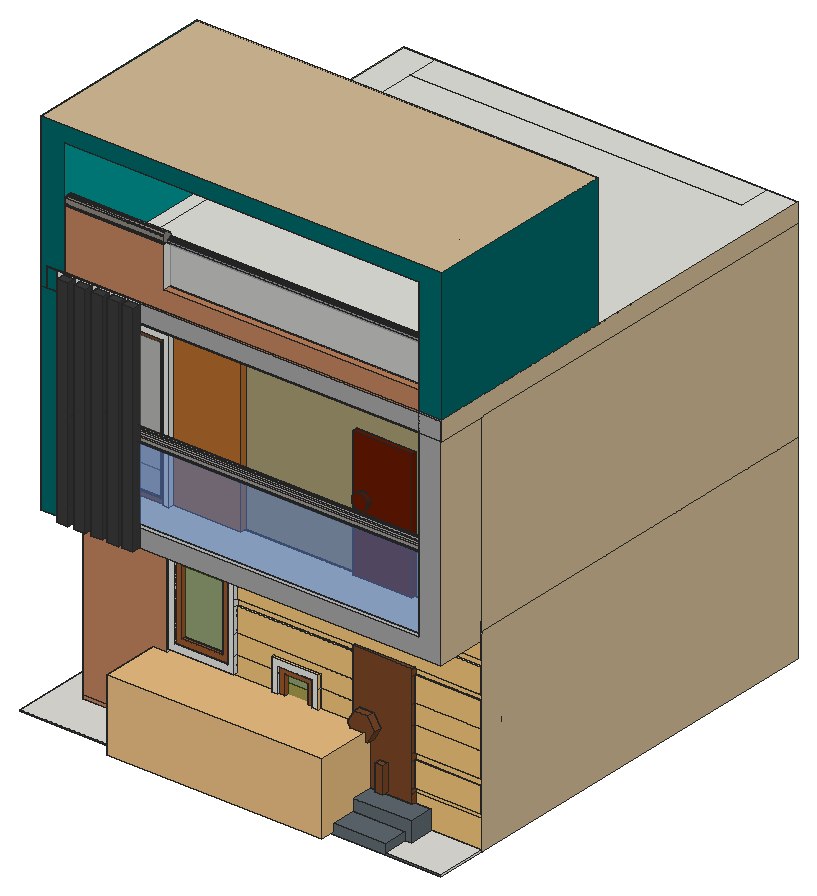
# SketchUp Ruby script. Lengths in inches.
U = 1.inch
M = Sketchup.active_model
def pt(a) = Geom::Point3d.new(a.map { |v| v * U })
def face(e, loops, mat)
  f = e.add_face(loops[0].map { |a| pt(a) })
  loops[1..].each { |l| e.add_face(l.map { |a| pt(a) }).erase! }
  f.material = f.back_material = mat if mat
  f
end
# faces: each face lists its corners as indices into pts; further lists are holes
def faces(e, pts, list, mat = nil) = list.each { |f| face(e, (f[0].is_a?(Array) ? f : [f]).map { |l| l.map { |i| pts[i] } }, mat) }
# xy, xz, yz: faces in a plane at the given z, y or x. An outline is a flat list of corners, or four numbers for a rectangle; further outlines are holes
def ring(l) = l.size == 4 ? [[l[0], l[1]], [l[2], l[1]], [l[2], l[3]], [l[0], l[3]]] : l.each_slice(2).to_a
def flat(e, list, mat, &to3) = list.each { |f| face(e, (f[0].is_a?(Array) ? f : [f]).map { |l| ring(l).map { |u, v| to3.(u, v) } }, mat) }
def xy(e, z, list, mat = nil) = flat(e, list, mat) { |x, y| [x, y, z] }
def xz(e, y, list, mat = nil) = flat(e, list, mat) { |x, z| [x, y, z] }
def yz(e, x, list, mat = nil) = flat(e, list, mat) { |y, z| [x, y, z] }
def lines(e, pts, list) = list.each { |a, b| e.add_line(pt(pts[a]), pt(pts[b])) }
# prism: a flat outline (further loops are holes) pulled along v
def prism(e, loops, v, mat = nil)
  f = face(e, loops, mat); d = Geom::Vector3d.new(v.map { |x| x * U })
  f.pushpull(f.normal.samedirection?(d) ? d.length : -d.length)
end
def box(e, o, s, mat = nil) = prism(e, [[o, [o[0] + s[0], o[1], o[2]], [o[0] + s[0], o[1] + s[1], o[2]], [o[0], o[1] + s[1], o[2]]]], [0, 0, s[2]], mat)
def at(x, y, z, deg = 0) = Geom::Transformation.translation(pt([x, y, z])) * Geom::Transformation.rotation(ORIGIN, Z_AXIS, deg.degrees)
def axes(o, x, y, z) = Geom::Transformation.new([*x, 0, *y, 0, *z, 0, *pt(o).to_a, 1])
def part(name) = M.definitions.add(name)
# library, detail: a bought-in or finely detailed component or shape, given as its bounding box
def library(name, o, s) = part(name).tap { |d| box(d.entities, o, s) }
def detail(e, o, s) = box(e.add_group.entities, o, s)
def put(e, d, t, mat = nil) = e.add_instance(d, t).tap { |i| i.material = mat if mat }
def group(e, t, mat = nil) = e.add_group.tap { |g| g.transformation = t; g.material = mat if mat }.entities
root = M.entities
M.materials.add("[Basic Tile]").color = [203, 206, 202]
M.materials.add("[Blacktop Old 01]").color = [132, 136, 139]
M.materials.add("[Color B08]").color = [102, 25, 0]
M.materials.add("[Color H07]").color = [0, 153, 153]
M.materials.add("[Color H08]").color = [0, 102, 102]
M.materials.add("[Color M07]").color = [58, 58, 58]
M.materials.add("[Concrete Aggregate Smoke]").color = [154, 150, 148]
M.materials.add("[Concrete Scored Jointless]").color = [140, 133, 127]
M.materials.add("[Concrete Tile]").color = [203, 190, 164]
M.materials.add("[Formica Beige]").color = [211, 187, 149]
M.materials.add("[Formica Speckled Grey]").color = [94, 105, 111]
M.materials.add("[Marble Carrara Gold Floor Tile]").color = [225, 223, 217]
M.materials.add("[Mirror 01]").color = [185, 185, 185]
M.materials.add("[Pavers Flagstone Gray]").color = [162, 162, 162]
M.materials.add("[Quartz Light Brown]").color = [199, 184, 152]
M.materials.add("[Terrazzo Light Blue]").color = [196, 214, 227]
M.materials.add("[Translucent Glass Blue]").color = [100, 149, 237]
M.materials["[Translucent Glass Blue]"].alpha = 0.5
M.materials.add("[Translucent Glass Dark Green]").color = [62, 91, 5]
M.materials["[Translucent Glass Dark Green]"].alpha = 0.5
M.materials.add("[Translucent Glass Gray]").color = [128, 128, 128]
M.materials["[Translucent Glass Gray]"].alpha = 0.5
M.materials.add("[Translucent Resin Crush Gray]").color = [184, 184, 184]
M.materials["[Translucent Resin Crush Gray]"].alpha = 0.8
M.materials.add("[Water Stream Shallow]").color = [155, 145, 133]
M.materials.add("[Wood Bamboo]").color = [177, 105, 43]
M.materials.add("[Wood Cherry Original]").color = [152, 86, 42]
M.materials.add("[Wood Floor Parquet]").color = [145, 89, 39]
M.materials.add("[Wood Lumber ButtJoined]").color = [164, 152, 112]
M.materials.add("[Wood OSB]").color = [240, 195, 122]
M.materials.add("[Wood Veneer 01]").color = [120, 70, 37]
M.materials.add("[Wood Veneer 02]").color = [190, 128, 91]
c1 = library("SHRUB",[-13.14,-8.45,-0.125],[75.37,32.45,24.02])
xy(root,0,[[0,4.95,16.1875,276],[16.1875,4.95,16.1875,276,16.63,276,16.63,32,67.83,32,67.83,35,180.1,35,180.1,33,216.1,33,216.1,36,256.1875,36,256.1875,4.95],[16.63,32,67.83,32,67.83,35,180.1,35,180.1,33,216.1,33,216.1,36,16.63,36],[16.63,36,256.1875,36,256.1875,244.95,247.63,244.95,247.63,45,25.63,45,25.63,244.95,16.63,244.95],[256.1875,36,256.1875,244.95,247.63,244.95,247.63,267,25.63,267,25.63,244.95,16.63,244.95,16.63,276,256.63,276,256.63,36],
  [25.63,45,247.63,244.95],[25.63,244.95,247.63,267]])
xy(root,1,[[173.84,20,173.84,35,180.1,35,180.1,33,216.1,33,216.1,35,226.28,35,226.28,20],[180.1,33,216.1,35]])
xy(root,1,[[0,4.95,173.84,4.95,173.84,35,67.83,35,67.83,32,16.63,32,16.63,276,0,276],[222.44,4.95,256.1875,4.95,256.1875,36,216.1,36,216.1,35,226.28,35,226.28,20,222.44,20]],"[Marble Carrara Gold Floor Tile]")
xy(root,3,[[16.63,32,67.83,36],[180.1,33,216.1,36],[67.83,35,151.74,36],[151.74,35,155.4,36],[155.4,35,159.06,36],
  [159.06,35,180.1,36],[67.83,36,151.74,39.4375],[151.74,36,155.4,39.4375],[155.4,36,159.06,39.4375],[159.06,36,180.1,39.4375]])
xy(root,6,[[173.84,4.95,222.44,20]],"[Formica Speckled Grey]")
xy(root,13,[[173.84,20,226.28,20,226.28,35,216.1,35,216.1,33,180.1,33,180.1,35,173.84,35]],"[Formica Speckled Grey]")
xy(root,14.41,[[196.71,29,201.46,33]])
xy(root,18.18,[[67.83,36,180.1,39.4375]])
xy(root,18.18,[[67.83,35,180.1,36]],"[Wood OSB]")
xy(root,19.49,[[130.75,33,159.06,36]],"[Wood OSB]")
xy(root,20.95,[[67.83,35,71.65,36],[71.65,35,75.54,36],[216.1,35,256.63,36],[159.06,36,180.1,40]])
xy(root,20.95,[[75.54,35,130.75,36],[159.06,35,180.1,36]],"[Wood OSB]")
xy(root,23.14,[[134.4,33,155.4,34],[134.4,34,155.4,36]])
xy(root,26.81,[[138.07,34,151.74,36]],"[Wood Cherry Original]")
xy(root,30.34,[[196.71,29,201.46,33]],"[Wood Veneer 01]")
xy(root,36.125,[[216.1,35,256.63,36],[159.06,36,180.1,40]])
xy(root,36.125,[[67.83,35,71.65,36],[71.65,35,75.54,36],[75.54,35,99.82,36],[99.82,35,100.35,36],[100.35,35,130.75,36],
  [159.06,35,180.1,36]],"[Wood OSB]")
xy(root,39.89,[[184.28,29,192.79,33]],"[Wood Veneer 01]")
xy(root,40.26,[[67.83,35,71.65,36],[71.65,35,75.54,36],[216.1,35,256.63,36]])
xy(root,40.26,[[75.54,35,130.75,36],[159.06,35,180.1,36]],"[Wood OSB]")
xy(root,45.68,[[67.83,33,108.0625,35],[67.83,35,108.0625,36]])
xy(root,49.49,[[71.65,33,104.25,34],[71.65,34,104.25,36]])
xy(root,53.39,[[75.54,34,100.35,36]],"[Wood Cherry Original]")
xy(root,54.64,[[184.28,29,192.79,33]],"[Wood Veneer 01]")
xy(root,55.4375,[[108.0625,35,130.75,36],[159.06,35,180.1,36],[216.1,35,256.63,36]])
xy(root,56.04,[[138.07,34,151.74,36]],"[Wood Cherry Original]")
xy(root,59.71,[[134.4,33,155.4,34],[134.4,34,155.4,36]])
xy(root,63.36,[[130.75,35,159.06,36]])
xy(root,63.36,[[130.75,33,159.06,35]],"[Wood OSB]")
xy(root,67.32,[[108.0625,35,180.1,36],[216.1,35,256.63,36]])
xy(root,82.5,[[108.0625,35,180.1,36],[216.1,35,256.63,36]])
xy(root,86.2,[[108.0625,35,180.1,36],[216.1,35,256.63,36]])
xy(root,87,[[180.1,35,216.1,36]])
xy(root,87,[[180.1,33,216.1,35]],"[Wood Veneer 01]")
xy(root,93.53,[[75.54,34,100.35,36]],"[Wood Cherry Original]")
xy(root,97.43,[[71.65,33,104.25,34],[71.65,34,104.25,36]])
xy(root,101.24,[[67.83,33,108.0625,35],[67.83,35,108.0625,36]])
xy(root,101.375,[[67.83,35,99.82,36],[99.82,35,180.1,36],[180.1,35,216.1,36],[216.1,35,256.63,36]])
xy(root,104.82,[[67.83,35,256.63,36]])
xy(root,114.54,[[72.76,5,256.15,35],[67.83,35,254.58,44]])
xy(root,114.54,[[36.83,0,36.83,5,12.82,5,12.82,32,67.83,32,67.83,35,72.76,35,72.76,5,43.69,5,43.69,0]],"[Color H07]")
xy(root,114.54,[[26.39,0,33.26,2],[47.39,0,54.26,5],[57.02,0,63.88,5],[65.89,0,72.76,5],[26.39,2,33.26,5]],"[Color M07]")
xy(root,117,[[25.63,45,247.63,267]])
xy(root,120,[[180.1,33,216.1,35],[67.83,35,99.82,36],[99.82,35,180.1,36],[180.1,35,216.1,36],[216.1,35,256.63,36]])
xy(root,125.64,[[25.76,5,36.83,8],[41.16,29,44.89,32],[67.83,29,71.5625,32],[44.89,30,67.83,32],[67.83,32,112.88,35],
  [67.83,35,112.88,36],[242.55,35,254.58,35.75],[254.58,35,256.15,35.75]])
xy(root,125.64,[[25.76,8,242.55,8,242.55,35,112.88,35,112.88,32,71.5625,32,71.5625,29,67.83,29,67.83,30,44.89,30,44.89,29,41.16,29,41.16,32,25.76,32],[112.88,35,242.55,35,242.55,35.75,254.58,35.75,254.58,44,67.83,44,67.83,36,112.88,36]],"[Basic Tile]")
xy(root,125.64,[[12.82,32,16.63,36]],"[Color H08]")
xy(root,125.64,[[43.69,5,242.55,8]],"[Mirror 01]")
xy(root,127.71,[[46.96,30,65.76,32]],"[Wood Veneer 01]")
xy(root,204,[[180.1,33,216.1,36]],"[Color B08]")
xy(root,213.66,[[46.96,30,65.76,32]],"[Wood Veneer 01]")
xy(root,215.73,[[44.89,29,67.83,30],[44.89,30,67.83,32]])
xy(root,219.46,[[41.16,29,71.5625,32]])
xy(root,236.32,[[12.82,5,22.32,8],[12.82,8,12.82,35.75,16.63,35.75,16.63,32,22.32,32,22.32,8],[16.63,32,22.32,35.75],[22.32,32,112.88,35.75],[12.82,35.75,16.63,36],
  [16.63,35.75,22.32,36],[22.32,35.75,112.88,36],[12.82,36,16.63,123.625],[16.63,36,22.32,123.625]])
xy(root,236.32,[[25.76,8,25.76,32,112.88,32,112.88,35.75,242.55,35.75,242.55,8]],"[Wood Floor Parquet]")
xy(root,237,[[16.63,5,25.76,36],[16.63,36,256.63,276]])
xy(root,237,[[26.39,5,99.82,36],[99.82,5,256.63,36]],"[Wood Floor Parquet]")
xy(root,237.45,[[25.76,5,26.39,36]])
xy(root,247.45,[[26.39,0,33.26,5],[36.83,0,43.69,8],[47.39,0,54.26,5],[57.02,0,63.88,5],[65.89,0,72.76,5]],"[Color M07]")
xy(root,248.02,[[16.63,5,22.32,8],[22.32,5,242.55,8],[242.55,5,256.15,8],[16.63,8,256.15,35.75],[16.63,35.75,22.32,123.625]])
xy(root,249,[[16.63,5,22.32,8],[22.32,5,27.38,8],[27.38,5,242.55,10.02],[242.55,5,256.63,123.6],[16.63,8,27.38,35.75],
  [27.38,10.02,237.59,10.02,237.59,24.04,35.67,24.04,35.67,121.625,27.38,121.625],[237.59,10.02,242.55,10.02,242.55,123.6,256.63,123.6,256.63,276,237.59,276,237.59,256.96,35.67,256.96,35.67,123.625,102.26,123.625,102.26,121.625,35.67,121.625,35.67,24.04,237.59,24.04],[16.63,35.75,22.32,123.625],[22.32,35.75,27.38,123.625],[27.38,121.625,35.67,123.625],
  [35.67,121.625,102.26,123.625],[16.63,123.625,35.67,276],[35.67,256.96,237.59,276]])
xy(root,260.27,[[87.26,5,242.55,10.02]],"[Wood Veneer 02]")
xy(root,285,[[27.38,5,87.26,7.13],[27.38,7.13,87.26,8],[87.26,7.64,242.55,10.02],[242.55,7.64,250.64,10.02],[27.38,8,87.26,10.02]])
xy(root,305.31,[[46.08,117.4375,84.2,120.4375],[46.08,120.4375,84.2,121.625]])
xy(root,306.9,[[47.67,120.4375,82.61,121.625]])
xy(root,306.9,[[47.67,117.4375,82.61,120.4375]],"[Terrazzo Light Blue]")
xy(root,312.03,[[47.67,117.4375,82.61,120.4375],[47.67,120.4375,82.61,121.625]])
xy(root,313.62,[[46.08,117.4375,84.2,120.4375],[46.08,120.4375,84.2,121.625]])
xy(root,319.63,[[27.38,121.625,102.26,123.625]])
xy(root,319.63,[[27.38,5,27.38,121.625,102.26,121.625,102.26,123.625,242.55,123.625,242.55,5]],"[Concrete Tile]")
xy(root,329.2,[[12.82,5,256.63,5,256.63,123.6,242.55,123.6,242.55,123.625,12.82,123.625]],"[Formica Beige]")
xz(root,0,[[26.39,114.54,33.26,247.45],[36.83,114.54,43.69,247.45],[47.39,114.54,54.26,247.45],[57.02,114.54,63.88,247.45],[65.89,114.54,72.76,247.45]],"[Color M07]")
xz(root,4.95,[[0,0,256.1875,0,256.1875,1,222.44,1,222.44,6,173.84,6,173.84,1,0,1]],"[Formica Speckled Grey]")
xz(root,5,[[26.39,114.54,33.26,125.64],[47.39,114.54,54.26,125.64],[57.02,114.54,63.88,125.64],[65.89,114.54,72.76,125.64],[26.39,125.64,33.26,237],
  [47.39,125.64,54.26,237],[57.02,125.64,63.88,237],[65.89,125.64,72.76,237],[22.32,237,25.76,237,25.76,237.45,26.39,237.45,26.39,247.45,33.26,247.45,33.26,237.45,72.76,237.45,72.76,248.02,22.32,248.02],[26.39,237,33.26,237.45],
  [33.26,237,36.83,237.45],[36.83,237,43.69,237.45],[43.69,237,47.39,237.45],[47.39,237,54.26,237.45],[54.26,237,57.02,237.45],
  [57.02,237,63.88,237.45],[63.88,237,65.89,237.45],[65.89,237,72.76,237.45],[72.76,237,242.55,237.45],[26.39,237.45,33.26,247.45],
  [26.39,237.45,33.26,247.45],[47.39,237.45,54.26,247.45],[57.02,237.45,63.88,247.45],[65.89,237.45,72.76,247.45]])
xz(root,5,[[12.82,114.54,26.39,114.54,26.39,125.64,25.76,125.64,25.76,237,22.32,237,22.32,236.32,12.82,236.32],[33.26,114.54,36.83,125.64],[43.69,114.54,47.39,125.64],[54.26,114.54,57.02,125.64],[63.88,114.54,65.89,125.64],
  [12.82,236.32,22.32,236.32,22.32,237,16.63,237,16.63,249,27.38,249,27.38,319.63,242.55,319.63,242.55,249,256.63,249,256.63,329.2,12.82,329.2],[16.63,237,22.32,248.02]],"[Color H08]")
xz(root,5,[[27.38,286.39,87.26,289.59]],"[Concrete Scored Jointless]")
xz(root,5,[[72.76,114.54,256.15,114.54,256.15,237,242.55,237,242.55,125.64,72.76,125.64],[242.55,237,256.15,248.02],[256.15,237,256.63,237,256.63,249,242.55,249,242.55,248.02,256.15,248.02],[72.76,237.45,242.55,248.02]],"[Pavers Flagstone Gray]")
xz(root,5,[[16.63,248.02,242.55,249],[27.38,249,242.55,249,242.55,260.27,87.26,260.27,87.26,285,27.38,285]],"[Wood Veneer 02]")
xz(root,8,[[36.83,125.64,43.69,139.27],[36.83,139.27,43.69,169.76],[36.83,169.76,43.69,170.73],[25.76,170.73,36.83,172.92],[36.83,170.73,43.69,172.92],
  [36.83,172.92,43.69,236.32],[36.83,236.32,43.69,247.45],[16.63,248.02,22.32,249]])
xz(root,8,[[25.76,125.64,36.83,169.76]],"[Color M07]")
xz(root,8,[[43.69,170.73,242.55,172.92]],"[Concrete Aggregate Smoke]")
xz(root,8,[[43.69,125.64,242.55,169.76]],"[Translucent Glass Blue]")
xz(root,10.02,[[27.38,249,27.38,285,87.26,285,87.26,260.27,237.59,260.27,237.59,249],[237.59,249,242.55,260.27],[242.55,282.625,250.64,285]])
xz(root,10.02,[[87.26,260.27,242.55,285]],"[Translucent Resin Crush Gray]")
xz(root,20,[[173.84,1,222.44,6]])
xz(root,20,[[222.44,1,226.28,1,226.28,13,173.84,13,173.84,6,222.44,6]],"[Formica Speckled Grey]")
xz(root,29,[[41.16,125.64,44.89,125.64,44.89,215.73,67.83,215.73,67.83,125.64,71.5625,125.64,71.5625,219.46,41.16,219.46]])
xz(root,29,[[196.71,14.41,201.46,30.34],[184.28,39.89,192.79,39.89,197.05,47.27,192.79,54.64,184.28,54.64,180.1,47.41,180.1,47.125]],"[Wood Veneer 01]")
xz(root,30,[[186.86,163.78,188.06,164.03,189.15,164.59,190.0625,165.4,190.73,166.43,191.11,167.59,191.18,168.81,190.93,170.01,190.38,171.1,189.5625,172.01,188.54,172.68,187.38,173.0625,186.16,173.13,184.96,172.88,183.87,172.33,182.95,171.51,182.28,170.49,181.9,169.33,181.83,168.11,182.08,166.91,182.63,165.82,183.45,164.9,184.47,164.23,185.64,163.85]],"[Color B08]")
xz(root,30,[[[44.89,125.64,67.83,215.73],[46.96,127.71,65.76,213.66]]],"[Wood Veneer 01]")
xz(root,32,[[16.63,0,67.83,1],[16.63,114.54,67.83,114.54,67.83,121.91,41.16,121.91,41.16,125.64,16.63,125.64],[41.16,121.91,67.83,125.64],[67.83,121.91,71.5625,125.64],[16.63,125.64,25.76,139.3125],
  [41.16,125.64,41.16,219.46,71.5625,219.46,71.5625,125.64,67.83,125.64,67.83,215.73,44.89,215.73,44.89,125.64],[[44.89,125.64,67.83,215.73],[46.96,127.71,65.76,213.66]],[16.63,139.3125,25.76,236.32]])
xz(root,32,[[12.82,114.54,16.63,125.64]],"[Color H08]")
xz(root,32,[[46.96,127.71,65.76,213.66]],"[Translucent Glass Gray]")
xz(root,32,[[25.76,125.64,41.16,125.64,41.16,219.46,71.5625,219.46,71.5625,125.64,112.88,125.64,112.88,236.32,25.76,236.32]],"[Wood Bamboo]")
xz(root,32,[[16.63,1,67.83,3],[16.63,3,67.83,114.54]],"[Wood Veneer 02]")
xz(root,33,[[180.1,0,216.1,1],[180.1,1,216.1,3],[180.1,3,216.1,13],[196.71,14.41,201.46,30.34],[[130.75,19.49,159.06,63.36],[134.4,23.14,155.4,59.71]],
  [184.28,39.89,180.1,47.125,180.1,47.41,184.28,54.64,192.79,54.64,197.05,47.27,192.79,39.89],[[67.83,45.68,108.0625,101.24],[71.65,49.49,104.25,97.43]],[180.1,47.125,180.1,47.41,180.02,47.27],[186.86,163.78,185.64,163.85,184.47,164.23,183.45,164.9,182.63,165.82,182.08,166.91,181.83,168.11,181.9,169.33,182.28,170.49,182.95,171.51,183.87,172.33,184.96,172.88,186.16,173.13,187.38,173.0625,188.54,172.68,189.5625,172.01,190.38,171.1,190.93,170.01,191.18,168.81,191.11,167.59,190.73,166.43,190.0625,165.4,189.15,164.59,188.06,164.03]])
xz(root,33,[[[180.1,120,216.1,204],[186.86,163.78,185.64,163.85,184.47,164.23,183.45,164.9,182.63,165.82,182.08,166.91,181.83,168.11,181.9,169.33,182.28,170.49,182.95,171.51,183.87,172.33,184.96,172.88,186.16,173.13,187.38,173.0625,188.54,172.68,189.5625,172.01,190.38,171.1,190.93,170.01,191.18,168.81,191.11,167.59,190.73,166.43,190.0625,165.4,189.15,164.59,188.06,164.03]]],"[Color B08]")
xz(root,33,[[[180.1,13,216.1,13,216.1,87,180.1,87,180.1,47.41,184.28,54.64,192.79,54.64,197.05,47.27,192.79,39.89,184.28,39.89,180.1,47.125],[196.71,14.41,201.46,30.34]]],"[Wood Veneer 01]")
xz(root,34,[[[134.4,23.14,155.4,59.71],[138.07,26.81,151.74,56.04]],[[71.65,49.49,104.25,97.43],[75.54,53.39,100.35,93.53]]],"[Wood Cherry Original]")
xz(root,35,[[67.83,0,151.74,1],[151.74,0,155.4,1],[155.4,0,159.06,1],[159.06,0,180.1,1],[173.84,1,180.1,3],
  [216.1,1,226.28,13],[173.84,3,180.1,13],[67.83,114.54,254.58,120],[254.58,114.54,256.15,120],[256.15,114.54,256.63,120],
  [67.83,120,254.58,125.64],[254.58,120,256.15,125.64]])
xz(root,35,[[67.83,1,173.84,3],[67.83,3,173.84,3,173.84,13,180.1,13,180.1,18.18,67.83,18.18],[67.83,20.95,130.75,36.125],[159.06,20.95,180.1,36.125],[216.1,20.95,256.63,36.125],
  [67.83,40.26,130.75,40.26,130.75,55.4375,108.0625,55.4375,108.0625,45.68,67.83,45.68],[159.06,40.26,180.1,55.4375],[216.1,40.26,256.63,55.4375],[108.0625,55.4375,130.75,55.4375,130.75,63.36,159.06,63.36,159.06,55.4375,180.1,55.4375,180.1,67.32,108.0625,67.32],[216.1,55.4375,256.63,67.32],
  [108.0625,67.32,180.1,82.5],[216.1,67.32,256.63,82.5],[108.0625,86.2,180.1,86.2,180.1,87,216.1,87,216.1,86.2,256.63,86.2,256.63,101.375,67.83,101.375,67.83,101.24,108.0625,101.24],[67.83,104.82,256.63,114.54]],"[Wood OSB]")
xz(root,35.75,[[242.55,125.64,242.55,236.32,22.32,236.32,22.32,248.02,256.15,248.02,256.15,125.64],[16.63,248.02,22.32,249]])
xz(root,36,[[16.63,0,216.1,3],[216.1,0,256.1875,1],[16.63,3,16.63,139.3125,112.88,139.3125,112.88,125.64,67.83,125.64,67.83,3],[67.83,3,180.1,18.18],[180.1,3,216.1,87],
  [[130.75,19.49,159.06,63.36],[134.4,23.14,155.4,59.71]],[67.83,20.95,130.75,36.125],[159.06,20.95,180.1,36.125],[216.1,20.95,256.63,36.125],[[134.4,23.14,155.4,59.71],[138.07,26.81,151.74,56.04]],
  [67.83,40.26,67.83,45.68,108.0625,45.68,108.0625,55.4375,130.75,55.4375,130.75,40.26],[159.06,40.26,180.1,55.4375],[216.1,40.26,256.63,55.4375],[[67.83,45.68,108.0625,101.24],[71.65,49.49,104.25,97.43]],[[71.65,49.49,104.25,97.43],[75.54,53.39,100.35,93.53]],
  [108.0625,55.4375,108.0625,67.32,180.1,67.32,180.1,55.4375,159.06,55.4375,159.06,63.36,130.75,63.36,130.75,55.4375],[216.1,55.4375,256.63,67.32],[108.0625,67.32,180.1,82.5],[216.1,67.32,256.63,82.5],[108.0625,86.2,108.0625,101.24,67.83,101.24,67.83,101.375,256.63,101.375,256.63,86.2,216.1,86.2,216.1,87,180.1,87,180.1,86.2],
  [67.83,104.82,256.63,120],[67.83,120,99.82,125.64],[180.1,120,216.1,204],[16.63,139.3125,112.88,236.32],[16.63,236.32,99.82,237],
  [25.76,237,26.39,237.45]])
xz(root,36,[[12.82,125.64,16.63,236.32]],"[Color H08]")
xz(root,36,[[138.07,26.81,151.74,56.04],[75.54,53.39,100.35,93.53]],"[Translucent Glass Dark Green]")
xz(root,36,[[99.82,120,180.1,120,180.1,204,216.1,204,216.1,120,256.63,120,256.63,237,99.82,237,99.82,236.32,112.88,236.32,112.88,125.64,99.82,125.64]],"[Wood Lumber ButtJoined]")
xz(root,36,[[256.1875,0,256.63,0,256.63,18.18,216.1,18.18,216.1,1,256.1875,1],[67.83,18.18,180.1,18.18,180.1,20.95,159.06,20.95,159.06,19.49,130.75,19.49,130.75,20.95,67.83,20.95],[216.1,18.18,256.63,20.95],[67.83,36.125,130.75,40.26],[159.06,36.125,180.1,40.26],
  [216.1,36.125,256.63,40.26],[108.0625,82.5,180.1,86.2],[216.1,82.5,256.63,86.2],[67.83,101.375,256.63,104.82]],"[Wood OSB]")
xz(root,39.4375,[[67.83,3,180.1,18.18]])
xz(root,40,[[159.06,20.95,180.1,36.125]])
xz(root,44,[[67.83,114.54,254.58,125.64]])
xz(root,45,[[25.63,0,247.63,117],[25.63,117,247.63,120],[25.63,120,247.63,237]])
xz(root,117.4375,[[[46.08,305.31,84.2,313.62],[47.67,306.9,82.61,312.03]]],"[Terrazzo Light Blue]")
xz(root,120.4375,[[[46.08,305.31,84.2,313.62],[47.67,306.9,82.61,312.03]]])
xz(root,121.625,[[[46.08,305.31,84.2,313.62],[47.67,306.9,82.61,312.03]]])
xz(root,121.625,[[[27.38,249,102.26,319.63],[46.08,305.31,84.2,313.62]]],"[Quartz Light Brown]")
xz(root,123.6,[[242.55,249,256.63,329.2]])
xz(root,123.625,[[12.82,236.32,12.82,329.2,27.38,329.2,27.38,249,16.63,249,16.63,248.02,22.32,248.02,22.32,236.32],[27.38,319.63,102.26,329.2],[102.26,319.63,242.55,329.2]])
xz(root,267,[[25.63,0,247.63,117],[25.63,117,247.63,120],[25.63,120,247.63,237]])
xz(root,276,[[0,0,16.63,1]])
xz(root,276,[[16.63,0,256.63,117],[16.63,117,256.63,120],[16.63,120,256.63,237],[16.63,237,256.63,249]],"[Formica Beige]")
yz(root,0,[[4.95,0,276,1]])
yz(root,12.82,[[5,114.54,5,236.32,36,236.32,36,125.64,32,125.64,32,114.54],[5,236.32,8,329.2],[8,236.32,35.75,329.2],[35.75,236.32,123.625,329.2]],"[Color H08]")
yz(root,16.63,[[32,0,36,1],[36,0,276,1],[32,1,36,3],[32,125.64,36,139.3125],[32,139.3125,36,236.32],
  [5,248.02,8,249],[8,248.02,35.75,249],[35.75,248.02,123.625,249]])
yz(root,16.63,[[36,1,276,237],[5,237,5,248.02,123.625,248.02,123.625,249,276,249,276,237]],"[Formica Beige]")
yz(root,16.63,[[32,3,36,125.64]],"[Wood Veneer 02]")
yz(root,22.32,[[5,236.32,8,248.02],[35.75,236.32,123.625,248.02]])
yz(root,25.63,[[45,0,267,117],[45,117,267,120],[45,120,267,237]])
yz(root,25.76,[[5,125.64,8,125.64,8,170.73,7.95,170.84,7.82,171.82,7.95,172.8125,8,172.92,8,236.32,6.2,237,5,237],[8,125.64,32,125.64,32,236.32,8,236.32,8,172.92,8.33,173.73,8.94,174.52,9.73,175.125,10.65,175.51,11.64,175.64,12.62,175.51,13.54,175.125,14.33,174.52,14.9375,173.73,15.32,172.8125,15.45,171.82,15.32,170.84,14.9375,169.92,14.33,169.13,13.54,168.52,12.62,168.14,11.64,168.01,10.65,168.14,9.73,168.52,8.94,169.13,8.33,169.92,8,170.73],[8,170.73,8,172.92,7.95,172.8125,7.82,171.82,7.95,170.84],[8,170.73,8,172.92,7.95,172.8125,7.82,171.82,7.95,170.84],[5,237,6.2,237,5,237.45],
  [6.2,237,36,237,36,237.45,5,237.45]])
yz(root,26.39,[[5,237,36,237.45]])
yz(root,26.39,[[0,114.54,5,247.45]],"[Color M07]")
yz(root,27.38,[[5,249,8,249,8,285,7.21,284.98,7.13,285,5,285],[8,249,10.02,285],[121.625,249,123.625,319.63],[7.21,284.98,8,285,7.13,285],[5,285,7.13,285,6.45,285.17,5.76,285.54,5.18,286.09,5,286.39],
  [5,286.39,5,289.59,4.72,289.07,4.53,288.3,4.55,287.51,4.77,286.76]])
yz(root,27.38,[[10.02,249,121.625,249,121.625,319.63,5,319.63,5,289.59,5.09,289.76,5.64,290.33,6.31,290.74,7.0625,290.96,7.85,290.98,8.62,290.8,9.31,290.42,9.88,289.875,10.29,289.2,10.51,288.45,10.53,287.66,10.35,286.9,9.97,286.2,9.43,285.63,8.76,285.22,8,285,10.02,285]],"[Color H07]")
yz(root,33.26,[[0,114.54,5,247.45]],"[Color M07]")
yz(root,36.83,[[5,125.64,8,139.27],[5,139.27,8,247.45]])
yz(root,36.83,[[0,114.54,5,139.27],[0,139.27,5,247.45]],"[Color M07]")
yz(root,41.16,[[29,125.64,32,219.46]])
yz(root,43.69,[[5,125.64,8,139.27],[5,139.27,8,247.45]])
yz(root,43.69,[[0,114.54,5,247.45]],"[Color M07]")
yz(root,44.89,[[29,125.64,30,215.73],[30,125.64,32,215.73]])
yz(root,46.08,[[117.4375,305.31,120.4375,313.62],[120.4375,305.31,121.625,313.62]])
yz(root,46.96,[[30,127.71,32,213.66]],"[Wood Veneer 01]")
yz(root,47.39,[[0,114.54,5,247.45]],"[Color M07]")
yz(root,47.67,[[117.4375,306.9,120.4375,312.03],[120.4375,306.9,121.625,312.03]])
yz(root,54.26,[[0,114.54,5,247.45]],"[Color M07]")
yz(root,57.02,[[0,114.54,5,247.45]],"[Color M07]")
yz(root,63.88,[[0,114.54,5,247.45]],"[Color M07]")
yz(root,65.76,[[30,127.71,32,213.66]],"[Wood Veneer 01]")
yz(root,65.89,[[0,114.54,5,247.45]],"[Color M07]")
yz(root,67.83,[[32,0,35,1],[32,1,35,3],[32,3,35,18.18],[35,3,36,18.18],[36,3,39.4375,18.18],
  [32,18.18,36,20.95],[32,20.95,35,36.125],[35,20.95,36,36.125],[32,36.125,36,40.26],[32,40.26,35,45.68],
  [35,40.26,36,45.68],[33,45.68,36,101.24],[35,101.24,36,101.375],[35,104.82,36,114.54],[32,114.54,35,125.64],
  [35,114.54,36,120],[36,114.54,44,125.64],[35,120,36,125.64],[29,125.64,30,215.73],[30,125.64,32,215.73]])
yz(root,67.83,[[32,45.68,33,45.68,33,101.24,35,101.24,35,101.375,36,101.375,36,104.82,35,104.82,35,114.54,32,114.54]],"[Wood Veneer 02]")
yz(root,71.5625,[[29,125.64,32,219.46]])
yz(root,71.65,[[33,49.49,34,97.43],[34,49.49,36,97.43]])
yz(root,72.76,[[0,114.54,5,247.45]],"[Color M07]")
yz(root,75.54,[[34,53.39,36,93.53]],"[Wood Cherry Original]")
yz(root,82.61,[[117.4375,306.9,120.4375,312.03],[120.4375,306.9,121.625,312.03]])
yz(root,84.2,[[117.4375,305.31,120.4375,313.62],[120.4375,305.31,121.625,313.62]])
yz(root,87.26,[[5,260.27,10.02,285],[10.02,282.625,10.02,285,8,285,8.76,285.22,9.43,285.63,9.97,286.2,10.35,286.9,10.45,287.32,10.63,287.29,11.2,287.06,11.7,286.68,12.07,286.1875,12.31,285.61,12.39,285,12.31,284.39,12.07,283.8125,11.7,283.32,11.2,282.94,10.63,282.71],[7.64,285,8,285,8.76,285.22,9.43,285.63,9.97,286.2,10.35,286.9,10.45,287.32,10.02,287.375,9.4,287.29,8.83,287.06,8.34,286.68,7.96,286.1875,7.72,285.61]])
yz(root,87.26,[[7.13,285,7.64,285,7.72,285.61,7.96,286.1875,8.34,286.68,8.83,287.06,9.4,287.29,10.02,287.375,10.45,287.32,10.53,287.66,10.51,288.45,10.29,289.2,9.88,289.875,9.31,290.42,8.62,290.8,7.85,290.98,7.0625,290.96,6.31,290.74,5.64,290.33,5.09,289.76,5,289.59,5,286.39,5.18,286.09,5.76,285.54,6.45,285.17]],"[Concrete Scored Jointless]")
yz(root,100.35,[[34,53.39,36,93.53]],"[Wood Cherry Original]")
yz(root,102.26,[[121.625,249,123.625,319.63]])
yz(root,104.25,[[33,49.49,34,97.43],[34,49.49,36,97.43]])
yz(root,108.0625,[[33,45.68,35,55.4375],[35,45.68,36,55.4375],[33,55.4375,35,67.32],[35,55.4375,36,67.32],[33,67.32,35,82.5],
  [35,67.32,36,82.5],[33,82.5,36,86.2],[33,86.2,35,101.24],[35,86.2,36,101.24]])
yz(root,112.88,[[32,125.64,36,236.32]],"[Wood Bamboo]")
yz(root,130.75,[[35,20.95,36,36.125],[35,40.26,36,55.4375],[35,55.4375,36,63.36]])
yz(root,130.75,[[33,19.49,36,20.95],[33,20.95,35,36.125],[33,36.125,36,40.26],[33,40.26,35,55.4375],[33,55.4375,35,63.36]],"[Wood OSB]")
yz(root,134.4,[[33,23.14,34,59.71],[34,23.14,36,59.71]])
yz(root,138.07,[[34,26.81,36,56.04]],"[Wood Cherry Original]")
yz(root,151.74,[[34,26.81,36,56.04]],"[Wood Cherry Original]")
yz(root,155.4,[[33,23.14,34,59.71],[34,23.14,36,59.71]])
yz(root,159.06,[[35,20.95,36,36.125],[36,20.95,40,36.125],[35,40.26,36,55.4375],[35,55.4375,36,63.36]])
yz(root,159.06,[[33,19.49,36,20.95],[33,20.95,35,36.125],[33,36.125,36,40.26],[33,40.26,35,55.4375],[33,55.4375,35,63.36]],"[Wood OSB]")
yz(root,173.84,[[4.95,1,20,6],[20,1,35,13]],"[Formica Speckled Grey]")
yz(root,180.1,[[33,0,35,1],[33,1,35,3],[33,3,35,13],[35,3,36,18.18],[36,3,39.4375,18.18],
  [35,20.95,36,36.125],[36,20.95,40,36.125],[35,40.26,36,55.4375],[35,55.4375,36,67.32],[35,67.32,36,82.5],
  [33,82.5,36,86.2],[33,86.2,35,87],[35,86.2,36,87]])
yz(root,180.1,[[33,120,36,204]],"[Color B08]")
yz(root,180.1,[[33,13,35,18.18],[33,18.18,36,20.95],[33,20.95,35,36.125],[33,36.125,36,40.26],[33,40.26,35,55.4375],
  [29,47.125,33,47.41],[33,55.4375,35,67.32],[33,67.32,35,82.5]],"[Wood Veneer 01]")
yz(root,196.71,[[29,14.41,33,30.34]],"[Wood Veneer 01]")
yz(root,201.46,[[29,14.41,33,30.34]],"[Wood Veneer 01]")
yz(root,216.1,[[33,0,36,1],[33,1,35,3],[35,1,36,3],[33,3,35,13],[35,20.95,36,36.125],
  [35,40.26,36,55.4375],[35,55.4375,36,67.32],[35,67.32,36,82.5],[35,86.2,36,87]])
yz(root,216.1,[[33,120,36,204]],"[Color B08]")
yz(root,216.1,[[35,3,36,3,36,18.18,33,18.18,33,13,35,13],[33,18.18,36,20.95],[33,20.95,35,36.125],[33,36.125,36,40.26],[33,40.26,35,55.4375],
  [33,55.4375,35,67.32],[33,67.32,35,82.5],[33,82.5,36,86.2],[33,86.2,35,87]],"[Wood Veneer 01]")
yz(root,222.44,[[4.95,1,20,6]],"[Formica Speckled Grey]")
yz(root,226.28,[[20,1,35,13]],"[Formica Speckled Grey]")
yz(root,242.55,[[5,249,10.02,260.27],[123.6,319.63,123.625,329.2]])
yz(root,242.55,[[[10.02,249,10.02,260.27,5,260.27,5,319.63,123.6,319.63,123.6,249],[10.02,282.625,10.63,282.71,11.2,282.94,11.7,283.32,12.07,283.8125,12.31,284.39,12.39,285,12.31,285.61,12.07,286.1875,11.7,286.68,11.2,287.06,10.63,287.29,10.02,287.375,9.4,287.29,8.83,287.06,8.34,286.68,7.96,286.1875,7.72,285.61,7.64,285,10.02,285]]],"[Color H07]")
yz(root,242.55,[[5,125.64,5,237.45,8,236.32,8,125.64],[8,125.64,8,170.73,8.33,169.92,8.94,169.13,9.73,168.52,10.65,168.14,11.64,168.01,12.62,168.14,13.54,168.52,14.33,169.13,14.9375,169.92,15.32,170.84,15.45,171.82,15.32,172.8125,14.9375,173.73,14.33,174.52,13.54,175.125,12.62,175.51,11.64,175.64,10.65,175.51,9.73,175.125,8.94,174.52,8.33,173.73,8,172.92,8,236.32,35.75,236.32,35.75,125.64]],"[Water Stream Shallow]")
yz(root,247.63,[[45,0,267,117],[45,117,267,120],[45,120,267,237]])
yz(root,250.64,[[10.02,282.625,10.02,285,7.64,285,7.72,285.61,7.96,286.1875,8.34,286.68,8.83,287.06,9.4,287.29,10.02,287.375,10.63,287.29,11.2,287.06,11.7,286.68,12.07,286.1875,12.31,285.61,12.39,285,12.31,284.39,12.07,283.8125,11.7,283.32,11.2,282.94,10.63,282.71]])
yz(root,254.58,[[35,114.54,44,125.64]])
yz(root,256.15,[[5,114.54,35,114.54,35,125.64,35.75,125.64,35.75,248.02,5,248.02]],"[Formica Beige]")
yz(root,256.1875,[[4.95,0,36,1]])
yz(root,256.63,[[35,20.95,36,36.125],[35,40.26,36,55.4375],[35,55.4375,36,67.32],[35,67.32,36,82.5],[35,86.2,36,101.375],
  [35,104.82,36,120]])
yz(root,256.63,[[5,249,123.6,329.2]],"[Color H08]")
yz(root,256.63,[[36,0,276,120],[36,120,276,237],[5,237,276,249]],"[Formica Beige]")
p = [[180.1,33,47.125],[184.28,33,39.89],[184.28,29,39.89],[180.1,29,47.125],[192.79,33,39.89],[197.05,33,47.27],
  [197.05,29,47.27],[192.79,29,39.89],[192.79,33,54.64],[192.79,29,54.64],[184.28,33,54.64],[180.1,33,47.41],
  [180.1,29,47.41],[184.28,29,54.64],[185.64,33,163.85],[186.86,33,163.78],[186.86,30,163.78],[185.64,30,163.85],
  [188.06,33,164.03],[188.06,30,164.03],[184.47,33,164.23],[184.47,30,164.23],[189.15,33,164.59],[189.15,30,164.59],
  [183.45,33,164.9],[183.45,30,164.9],[190.0625,33,165.4],[190.0625,30,165.4],[182.63,33,165.82],[182.63,30,165.82],
  [190.73,33,166.43],[190.73,30,166.43],[182.08,33,166.91],[182.08,30,166.91],[191.11,33,167.59],[191.11,30,167.59],
  [181.83,33,168.11],[181.83,30,168.11],[191.18,33,168.81],[191.18,30,168.81],[25.76,10.65,168.14],[25.76,11.64,168.01],
  [242.55,11.64,168.01],[242.55,10.65,168.14],[25.76,12.62,168.14],[242.55,12.62,168.14],[25.76,9.73,168.52],[242.55,9.73,168.52],
  [25.76,13.54,168.52],[242.55,13.54,168.52],[181.9,33,169.33],[181.9,30,169.33],[25.76,8.94,169.13],[242.55,8.94,169.13],
  [25.76,14.33,169.13],[242.55,14.33,169.13],[190.93,33,170.01],[190.93,30,170.01],[25.76,8.33,169.92],[242.55,8.33,169.92],
  [25.76,14.9375,169.92],[242.55,14.9375,169.92],[182.28,33,170.49],[182.28,30,170.49],[25.76,8,170.73],[242.55,8,170.73],
  [43.69,8,170.73],[36.83,8,170.73],[25.76,15.32,170.84],[242.55,15.32,170.84],[190.38,33,171.1],[190.38,30,171.1],
  [182.95,33,171.51],[182.95,30,171.51],[25.76,15.45,171.82],[242.55,15.45,171.82],[189.5625,33,172.01],[189.5625,30,172.01],
  [183.87,33,172.33],[183.87,30,172.33],[25.76,15.32,172.8125],[242.55,15.32,172.8125],[188.54,33,172.68],[188.54,30,172.68],
  [184.96,33,172.88],[184.96,30,172.88],[187.38,33,173.0625],[187.38,30,173.0625],[25.76,14.9375,173.73],[242.55,14.9375,173.73],
  [25.76,8.33,173.73],[25.76,8,172.92],[36.83,8,172.92],[43.69,8,172.92],[242.55,8,172.92],[242.55,8.33,173.73],
  [186.16,33,173.13],[186.16,30,173.13],[25.76,8.94,174.52],[242.55,8.94,174.52],[25.76,14.33,174.52],[242.55,14.33,174.52],
  [25.76,9.73,175.125],[242.55,9.73,175.125],[25.76,13.54,175.125],[242.55,13.54,175.125],[25.76,10.65,175.51],[242.55,10.65,175.51],
  [25.76,12.62,175.51],[242.55,12.62,175.51],[25.76,11.64,175.64],[242.55,11.64,175.64],[25.76,6.2,237],[25.76,8,236.32],
  [36.83,8,236.32],[43.69,8,236.32],[242.55,8,236.32],[242.55,5,237.45],[72.76,5,237.45],[65.89,5,237.45],
  [63.88,5,237.45],[57.02,5,237.45],[54.26,5,237.45],[47.39,5,237.45],[43.69,5,237.45],[36.83,5,237.45],
  [33.26,5,237.45],[26.39,5,237.45],[25.76,5,237.45],[242.55,10.63,282.71],[242.55,10.02,282.625],[250.64,10.02,282.625],
  [250.64,10.63,282.71],[87.26,10.63,282.71],[87.26,11.2,282.94],[242.55,11.2,282.94],[250.64,11.2,282.94],[87.26,11.7,283.32],
  [242.55,11.7,283.32],[250.64,11.7,283.32],[87.26,12.07,283.8125],[242.55,12.07,283.8125],[250.64,12.07,283.8125],[87.26,12.31,284.39],
  [242.55,12.31,284.39],[250.64,12.31,284.39],[87.26,12.39,285],[242.55,12.39,285],[250.64,12.39,285],[27.38,6.45,285.17],
  [27.38,7.13,285],[87.26,7.13,285],[87.26,6.45,285.17],[87.26,7.72,285.61],[87.26,7.64,285],[242.55,7.64,285],
  [242.55,7.72,285.61],[250.64,7.72,285.61],[250.64,7.64,285],[27.38,8,285],[27.38,8.76,285.22],[87.26,8.76,285.22],
  [87.26,8,285],[87.26,12.31,285.61],[242.55,12.31,285.61],[250.64,12.31,285.61],[27.38,5.76,285.54],[87.26,5.76,285.54],
  [27.38,9.43,285.63],[87.26,9.43,285.63],[27.38,5.18,286.09],[87.26,5.18,286.09],[87.26,7.96,286.1875],[242.55,7.96,286.1875],
  [250.64,7.96,286.1875],[27.38,9.97,286.2],[87.26,9.97,286.2],[87.26,12.07,286.1875],[242.55,12.07,286.1875],[250.64,12.07,286.1875],
  [27.38,5,286.39],[87.26,5,286.39],[87.26,8.34,286.68],[242.55,8.34,286.68],[250.64,8.34,286.68],[27.38,10.35,286.9],
  [87.26,10.35,286.9],[87.26,11.7,286.68],[242.55,11.7,286.68],[250.64,11.7,286.68],[87.26,8.83,287.06],[242.55,8.83,287.06],
  [250.64,8.83,287.06],[87.26,11.2,287.06],[242.55,11.2,287.06],[250.64,11.2,287.06],[27.38,10.53,287.66],[87.26,10.53,287.66],
  [87.26,10.45,287.32],[87.26,9.4,287.29],[242.55,9.4,287.29],[250.64,9.4,287.29],[87.26,10.63,287.29],[242.55,10.63,287.29],
  [250.64,10.63,287.29],[87.26,10.02,287.375],[242.55,10.02,287.375],[250.64,10.02,287.375],[27.38,10.51,288.45],[87.26,10.51,288.45],
  [27.38,10.29,289.2],[87.26,10.29,289.2],[27.38,9.88,289.875],[87.26,9.88,289.875],[27.38,5.09,289.76],[27.38,5,289.59],
  [87.26,5,289.59],[87.26,5.09,289.76],[27.38,5.64,290.33],[87.26,5.64,290.33],[27.38,9.31,290.42],[87.26,9.31,290.42],
  [27.38,6.31,290.74],[87.26,6.31,290.74],[27.38,8.62,290.8],[87.26,8.62,290.8],[27.38,7.0625,290.96],[87.26,7.0625,290.96],
  [27.38,7.85,290.98],[87.26,7.85,290.98],[315.04,-22.41,117],[315.04,-22.41,120],[26.39,2,125.64],[33.26,2,125.64],
  [242.55,35.75,319.63],[242.55,35.75,329.2]]
faces(root,p,[[0,1,2,3],[4,5,6,7],[5,8,9,6],[10,11,12,13]],"[Wood Veneer 01]")
faces(root,p,[[14,15,16,17],[15,18,19,16],[20,14,17,21],[18,22,23,19],[24,20,21,25],[22,26,27,23],[28,24,25,29],[26,30,31,27],
  [32,28,29,33],[30,34,35,31],[36,32,33,37],[34,38,39,35],[50,36,37,51],[38,56,57,39],[62,50,51,63],[56,70,71,57],
  [72,62,63,73],[70,76,77,71],[78,72,73,79],[76,82,83,77],[84,78,79,85],[82,86,87,83],[96,84,85,97],[86,96,97,87]],"[Color B08]")
faces(root,p,[[40,41,42,43],[41,44,45,42],[46,40,43,47],[44,48,49,45],[52,46,47,53],[48,54,55,49],[58,52,53,59],[54,60,61,55],
  [64,58,59,65,66,67],[60,68,69,61],[68,74,75,69],[74,80,81,75],[80,88,89,81],[90,91,92,93,94,95],[98,90,95,99],[88,100,101,89],
  [102,98,99,103],[100,104,105,101],[106,102,103,107],[104,108,109,105],[110,106,107,111],[108,110,111,109]],"[Concrete Aggregate Smoke]")
faces(root,p,[[112,113,114,115,116,117,118,119,120,121,122,123,124,125,126,127,128]],"[Wood Floor Parquet]")
faces(root,p,[[129,130,131,132],[135,129,132,136],[138,135,136,139],[141,138,139,142],[144,141,142,145],[147,144,145,148],[155,156,157,158],[164,147,148,165],
  [156,173,174,157],[178,164,165,179],[173,183,184,174],[188,178,179,189],[183,191,192,184],[194,188,189,195],[191,200,201,192],[203,194,195,204],
  [200,206,207,201],[206,203,204,207]])
faces(root,p,[[133,134,135,129],[134,137,138,135],[137,140,141,138],[140,143,144,141],[143,146,147,144],[153,154,155,156],[146,163,164,147],[172,153,156,173],
  [163,177,178,164],[182,172,173,183],[177,187,188,178],[190,182,183,191],[187,193,194,188],[199,190,191,200],[193,202,203,194],[205,199,200,206],
  [198,205,206,203,202]],"[Blacktop Old 01]")
faces(root,p,[[149,150,151,152],[159,160,161,162],[166,149,152,167],[160,168,169,161],[170,166,167,171],[168,175,176,169],[180,170,171,181],[175,185,186,176],
  [185,196,197,198,186],[196,208,209,197],[208,210,211,209],[210,212,213,211],[214,215,216,217],[218,214,217,219],[212,220,221,213],[222,218,219,223],
  [220,224,225,221],[226,222,223,227],[224,228,229,225],[228,226,227,229]],"[Concrete Scored Jointless]")
lines(root,p,[[230,231],[232,233],[234,235]])
put(root,c1,axes([82.32,9.85,1.1],[1.73745,0,0],[0,1.5795,0],[0,0,1.81643]))
